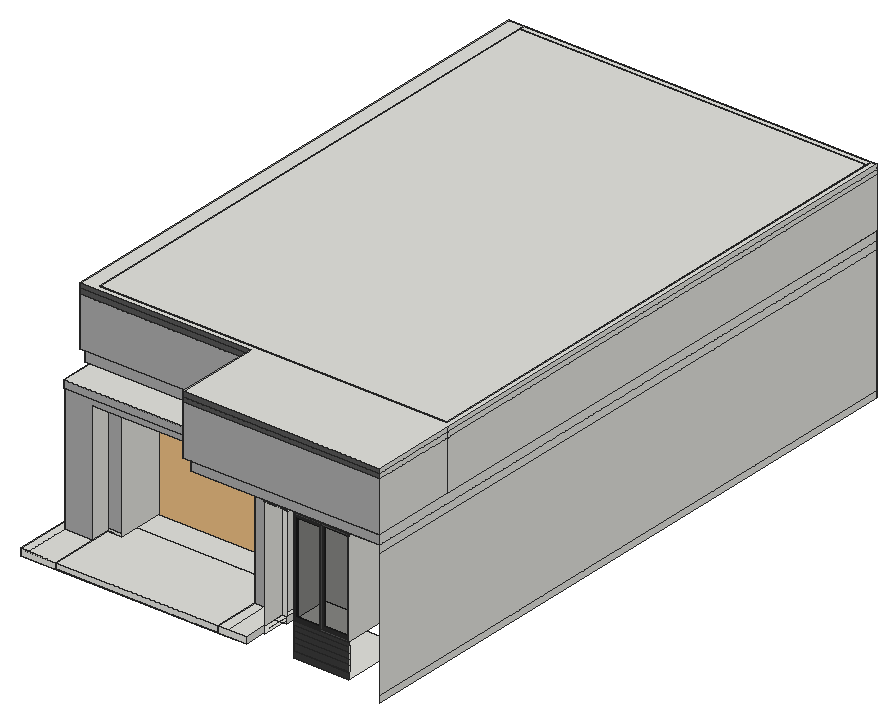
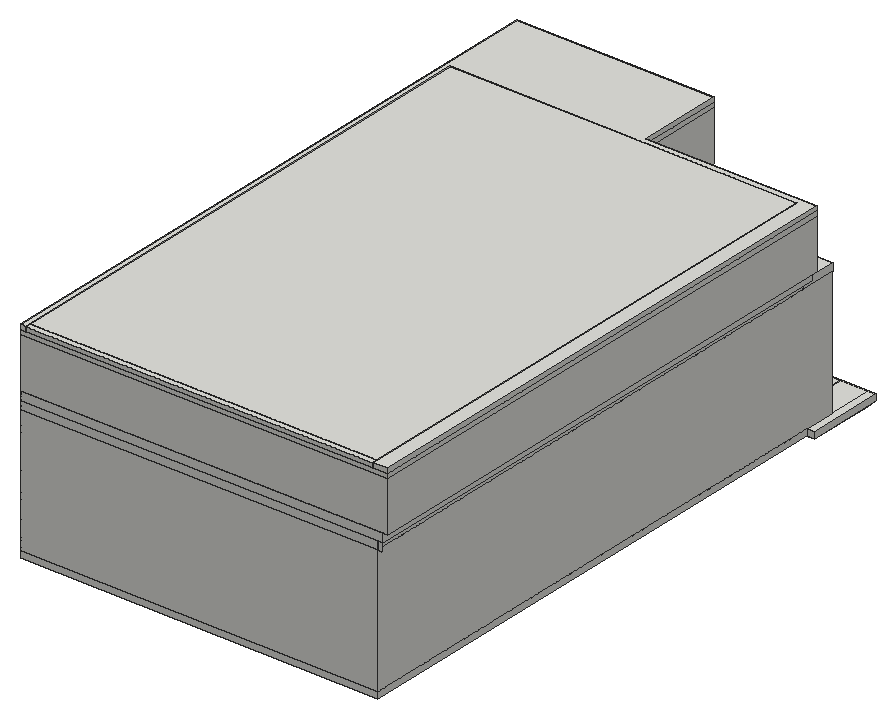
# SketchUp Ruby script. Lengths in inches.
U = 1.inch
M = Sketchup.active_model
def pt(a) = Geom::Point3d.new(a.map { |v| v * U })
def face(e, loops, mat)
  f = e.add_face(loops[0].map { |a| pt(a) })
  loops[1..].each { |l| e.add_face(l.map { |a| pt(a) }).erase! }
  f.material = f.back_material = mat if mat
  f
end
# faces: each face lists its corners as indices into pts; further lists are holes
def faces(e, pts, list, mat = nil) = list.each { |f| face(e, (f[0].is_a?(Array) ? f : [f]).map { |l| l.map { |i| pts[i] } }, mat) }
# xy, xz, yz: faces in a plane at the given z, y or x. An outline is a flat list of corners, or four numbers for a rectangle; further outlines are holes
def ring(l) = l.size == 4 ? [[l[0], l[1]], [l[2], l[1]], [l[2], l[3]], [l[0], l[3]]] : l.each_slice(2).to_a
def flat(e, list, mat, &to3) = list.each { |f| face(e, (f[0].is_a?(Array) ? f : [f]).map { |l| ring(l).map { |u, v| to3.(u, v) } }, mat) }
def xy(e, z, list, mat = nil) = flat(e, list, mat) { |x, y| [x, y, z] }
def xz(e, y, list, mat = nil) = flat(e, list, mat) { |x, z| [x, y, z] }
def yz(e, x, list, mat = nil) = flat(e, list, mat) { |y, z| [x, y, z] }
def lines(e, pts, list) = list.each { |a, b| e.add_line(pt(pts[a]), pt(pts[b])) }
# prism: a flat outline (further loops are holes) pulled along v
def prism(e, loops, v, mat = nil)
  f = face(e, loops, mat); d = Geom::Vector3d.new(v.map { |x| x * U })
  f.pushpull(f.normal.samedirection?(d) ? d.length : -d.length)
end
def box(e, o, s, mat = nil) = prism(e, [[o, [o[0] + s[0], o[1], o[2]], [o[0] + s[0], o[1] + s[1], o[2]], [o[0], o[1] + s[1], o[2]]]], [0, 0, s[2]], mat)
def at(x, y, z, deg = 0) = Geom::Transformation.translation(pt([x, y, z])) * Geom::Transformation.rotation(ORIGIN, Z_AXIS, deg.degrees)
def axes(o, x, y, z) = Geom::Transformation.new([*x, 0, *y, 0, *z, 0, *pt(o).to_a, 1])
def part(name) = M.definitions.add(name)
# library, detail: a bought-in or finely detailed component or shape, given as its bounding box
def library(name, o, s) = part(name).tap { |d| box(d.entities, o, s) }
def detail(e, o, s) = box(e.add_group.entities, o, s)
def put(e, d, t, mat = nil) = e.add_instance(d, t).tap { |i| i.material = mat if mat }
def group(e, t, mat = nil) = e.add_group.tap { |g| g.transformation = t; g.material = mat if mat }.entities
root = M.entities
M.materials.add("Glass_Tinted_Gray").color = [0, 0, 0]
M.materials["Glass_Tinted_Gray"].alpha = 0.125
M.materials.add("[0135_DarkGray]").color = [81, 81, 81]
M.materials.add("[Color M03]").color = [170, 170, 170]
M.materials.add("[Color M06]").color = [86, 86, 86]
M.materials.add("[Color M07]").color = [58, 58, 58]
M.materials.add("[Mirror 02]").color = [229, 229, 229]
M.materials.add("[Terrazzo Light Blue]").color = [196, 214, 227]
c1 = library("12",[112.18,111.43,0],[146.07,15.17,104.72])
c2 = part("PENTEK_RP Fineline 50S_Sliding_DoorCase_E1")
box(c2.entities,[0,0,0],[1.51,3.66,99.27],"[0135_DarkGray]")
c3 = part("PENTEK_RP Fineline 50S_SlidingDooe_Case_E2")
box(c3.entities,[0,0,0],[96.25,3.66,1.51],"[0135_DarkGray]")
c4 = part("pentek_RP Fineline 50S_SlidingDoor_Case")
put(c4.entities,c2,at(97.76,0,0))
put(c4.entities,c3,at(1.51,0,0))
put(c4.entities,c2,at(0,0,0))
put(c4.entities,c3,at(1.51,0,97.76))
c5 = part("PENTEK_RP Fineline 50S_SlidingDoor_GlazingBead_2")
box(c5.entities,[0,0,0],[0.56,0.59,94.39],"[0135_DarkGray]")
c6 = part("PENTEK_RP Fineline 50S_SlidingDoor_Glass")
box(c6.entities,[0,0,0],[46.58,0.16,94.39],"Glass_Tinted_Gray")
c7 = part("PENTEK_RP Fineline 50S_SlidingDoor_GlazingBead")
box(c7.entities,[0,0,0],[45.47,0.59,0.56],"[0135_DarkGray]")
c8 = part("PENTEK_RP Fineline 50S_SlidingDoor_Leaf_E1")
xy(c8.entities,0,[[0,0,0.93,1.97],[0.93,1.57,1.49,1.97]],"[0135_DarkGray]")
xy(c8.entities,96.25,[[0,0,0.93,0,0.93,1.57,1.49,1.57,1.49,1.97,0,1.97]],"[0135_DarkGray]")
xz(c8.entities,0,[[0,0,0.93,96.25]],"[0135_DarkGray]")
xz(c8.entities,1.57,[[0.93,0,1.49,95.32],[0.93,95.32,1.49,96.25]],"[0135_DarkGray]")
xz(c8.entities,1.97,[[0,0,1.49,96.25]],"[0135_DarkGray]")
yz(c8.entities,0,[[0,0,1.97,96.25]],"[0135_DarkGray]")
yz(c8.entities,0.93,[[0,0,1.57,0.93],[0,0.93,1.57,95.32],[0,95.32,1.57,96.25]],"[0135_DarkGray]")
yz(c8.entities,1.49,[[1.57,0,1.97,95.32],[1.57,95.32,1.97,96.25]],"[0135_DarkGray]")
c9 = part("PENTEK_RP Fineline 50S_SlidingDoor_Leaf_E2")
xy(c9.entities,0,[[0,0,0,1.57,0.56,1.57,0.56,1.97,46.02,1.97,46.02,1.57,46.58,1.57,46.58,0]],"[0135_DarkGray]")
xy(c9.entities,0.93,[[0,0,46.58,1.57]],"[0135_DarkGray]")
xy(c9.entities,1.49,[[0.56,1.57,46.02,1.97]],"[0135_DarkGray]")
xz(c9.entities,0,[[0,0,46.58,0.93]],"[0135_DarkGray]")
xz(c9.entities,1.57,[[0,0,0.56,0.93],[46.02,0,46.58,0.93],[0.56,0.93,46.02,1.49]],"[0135_DarkGray]")
xz(c9.entities,1.97,[[0.56,0,46.02,1.49]],"[0135_DarkGray]")
yz(c9.entities,0,[[0,0,1.57,0.93]],"[0135_DarkGray]")
yz(c9.entities,0.56,[[1.57,0,1.97,0.93],[1.57,0.93,1.97,1.49]],"[0135_DarkGray]")
yz(c9.entities,46.02,[[1.57,0,1.97,0.93],[1.57,0.93,1.97,1.49]],"[0135_DarkGray]")
yz(c9.entities,46.58,[[0,0,1.57,0.93]],"[0135_DarkGray]")
c10 = part("PENTEK_RP Fineline S_SlidingDoor_Leaf1")
put(c10.entities,c5,at(0.93,0,0.93))
put(c10.entities,c5,at(46.96,0,0.93))
put(c10.entities,c6,at(1.49,1.42,0.93))
put(c10.entities,c7,at(1.49,0,0.93))
put(c10.entities,c6,at(1.49,0.59,0.93),"[Terrazzo Light Blue]")
put(c10.entities,c8,at(0,0,0))
put(c10.entities,c8,axes([48.44,0,0],[-1,0,0],[0,1,0],[0,0,1]))
put(c10.entities,c9,axes([0.93,0,96.25],[1,0,0],[0,1,0],[0,0,-1]))
put(c10.entities,c9,at(0.93,0,0))
put(c10.entities,c7,at(1.49,0,94.77))
c11 = part("PENTEK_RP Fineline 50S_SlidingDoor_Leaf2")
put(c11.entities,c6,at(1.49,1.42,0.93))
put(c11.entities,c7,at(1.49,0,94.77))
put(c11.entities,c5,at(46.96,0,0.93))
put(c11.entities,c6,at(1.49,0.59,0.93),"[Mirror 02]")
put(c11.entities,c5,at(0.93,0,0.93))
put(c11.entities,c8,at(0,0,0))
put(c11.entities,c8,axes([48.44,0,0],[-1,0,0],[0,1,0],[0,0,1]))
put(c11.entities,c7,at(1.49,0,0.93))
put(c11.entities,c9,axes([0.93,0,96.25],[1,0,0],[0,1,0],[0,0,-1]))
put(c11.entities,c9,at(0.93,0,0))
c12 = part("PENTEK - Slimmest Steel Sliding Door / Window\#1")
put(c12.entities,c4,at(0,-1.88,-0.09))
put(c12.entities,c10,at(1.51,-2.27,1.42))
put(c12.entities,c11,at(49.32,-0.3,1.42))
c13 = library("Group\#72",[-0.5,-0.5,0],[113.04,13,1.125])
xy(root,246,[[184.16,507.49,380.7,517.74],[380.7,507.49,398.6,517.74],[184.16,517.74,189.35,580.49],[365.35,517.74,390.22,517.74,390.22,549.55,399.1,549.55,399.1,580.49,365.35,580.49],[390.22,517.74,398.6,517.74,398.6,528.52,399.1,528.52,399.1,549.55,390.22,549.55],
  [399.1,549.55,402.91,585.58],[365.35,580.49,399.1,585.58],[365.35,585.58,399.1,634.36]])
xy(root,246.1875,[[218.17,507.49,218.17,568.22,223.86,568.22,223.86,585.58,362.1,585.58,362.1,568.22,371.29,568.22,371.29,507.49]])
xy(root,246.25,[[439.12,512.52,491.67,577.96]])
xy(root,252,[[184.16,507.49,191.6,580.49],[191.6,507.49,218.17,550.86],[218.17,507.49,371.29,507.49,371.29,568.22,362.1,568.22,362.1,585.58,232.11,585.58,232.11,568.22,218.17,568.22],[371.29,507.49,380.7,550.86],[380.7,507.49,398.6,550.86],
  [398.6,528.52,398.66,549.55],[398.6,549.55,402.91,585.58],[371.29,550.86,380.7,631.58],[380.7,550.86,398.6,631.58],[223.86,568.22,232.11,585.58],
  [232.11,585.58,362.1,585.58,362.1,631.58,371.29,631.58,371.29,633.05,398.6,633.05,398.6,585.58,525.63,585.58,525.63,1083.4,196.6875,1083.4,196.6875,631.58,217.86,631.58,217.86,746.45,223.86,746.45,223.86,631.58,232.11,631.58],[217.86,631.58,223.86,746.45],[371.29,631.58,380.7,633.05],[380.7,631.58,398.6,633.05]])
xy(root,252.37,[[439.12,512.52,491.67,513.21]])
xy(root,274.3125,[[439.12,512.52,491.67,513.21]])
xy(root,278.25,[[439.12,512.52,491.67,549.55]])
xy(root,365.8125,[[[218.17,550.86,218.17,568.22,232.11,568.22,232.11,631.58,362.1,631.58,362.1,568.22,371.29,568.22,371.29,550.86],[347.6,562.2,349.15,562.4,350.6,563,351.84,563.96,352.79,565.2,353.39,566.65,353.6,568.2,353.39,569.75,352.79,571.2,351.84,572.44,350.6,573.4,349.15,574,347.6,574.2,346.04,574,344.6,573.4,343.35,572.44,342.4,571.2,341.8,569.75,341.6,568.2,341.8,566.65,342.4,565.2,343.35,563.96,344.6,563,346.04,562.4],[247.56,562.2,249.11,562.4,250.56,563,251.8,563.96,252.75,565.2,253.35,566.65,253.56,568.2,253.35,569.75,252.75,571.2,251.8,572.44,250.56,573.4,249.11,574,247.56,574.2,246,574,244.56,573.4,243.31,572.44,242.36,571.2,241.76,569.75,241.56,568.2,241.76,566.65,242.36,565.2,243.31,563.96,244.56,563,246,562.4],[299.84,562.2,301.39,562.4,302.84,563,304.08,563.96,305.04,565.2,305.64,566.65,305.84,568.2,305.64,569.75,305.04,571.2,304.08,572.44,302.84,573.4,301.39,574,299.84,574.2,298.29,574,296.84,573.4,295.6,572.44,294.64,571.2,294.04,569.75,293.84,568.2,294.04,566.65,294.64,565.2,295.6,563.96,296.84,563,298.29,562.4]],[362.1,568.22,371.29,585.58]])
xy(root,369.375,[[410.48,512.52,415.12,513.21],[415.12,512.52,416.48,528.52],[416.48,512.52,421.12,513.21],[421.12,512.52,422.48,528.52],[422.48,512.52,427.12,513.21],
  [427.12,512.52,428.48,528.52],[428.48,512.52,433.12,513.21],[433.12,512.52,434.48,528.52],[439.12,512.52,491.67,549.55]])
xy(root,372,[[191.6,549.55,398.6,550.86],[191.6,550.86,398.6,585.58],[196.6875,585.58,398.6,631.58]])
xy(root,375.375,[[410.48,512.52,497.28,528.52]])
xy(root,379.5625,[[515.78,500.24,515.78,580.49,501.41,580.49,501.41,585.58,525.63,585.58,525.63,1083.4,196.6875,1083.4,196.6875,585.58,191.6,585.58,191.6,1088.49,530.72,1088.49,530.72,500.24],[351.11,500.24,351.11,549.55,398.66,549.55,398.66,528.52,508.41,528.52,508.41,505.61,501.41,505.61,501.41,500.24],[501.41,500.24,501.41,505.61,513.53,505.61,513.53,502.86,508.41,502.86,508.41,500.24],[508.41,500.24,515.78,502.86],[513.53,502.86,513.53,521.24,508.41,521.24,508.41,580.49,515.78,580.49,515.78,502.86],
  [508.41,505.61,513.53,521.24],[398.66,528.52,402.91,549.55],[402.91,528.52,501.41,549.55],[501.41,528.52,508.41,580.49],[191.6,549.55,351.11,580.49],
  [351.11,549.55,501.41,585.58],[186.66,580.49,187.78,1088.49],[187.78,580.49,191.6,1088.49],[191.6,580.49,351.11,585.58]])
xy(root,388.5625,[[344.29,500.24,351.11,507.49],[351.11,500.24,530.72,580.49],[344.29,507.49,351.11,580.49],[182.47,580.49,186.66,1088.49],[[186.66,580.49,530.72,1088.49],[196.6875,585.58,525.63,1083.4]]])
xy(root,435.5,[[[344.29,500.24,344.29,580.49,182.47,580.49,182.47,1088.49,530.72,1088.49,530.72,500.24],[196.6875,585.58,525.63,1083.4]]])
xy(root,440.1875,[[344.29,500.24,344.29,580.49,182.47,580.49,182.47,1088.49,196.6875,1088.49,196.6875,585.58,525.63,585.58,525.63,1088.49,530.72,1088.49,530.72,500.24],[196.6875,585.58,525.63,1083.4],[196.6875,1083.4,525.63,1088.49]])
xy(root,444.75,[[344.29,500.24,530.72,500.24,530.72,1088.49,525.63,1088.49,525.63,585.58,196.6875,585.58,196.6875,1088.49,182.47,1088.49,182.47,580.49,344.29,580.49],[196.6875,585.58,525.63,1083.4],[196.6875,1083.4,525.63,1088.49]])
xz(root,500.24,[[351.11,379.5625,530.72,388.5625],[344.29,388.5625,530.72,435.5]],"[Color M03]")
xz(root,500.24,[[344.29,435.5,530.72,440.1875],[344.29,440.1875,530.72,444.75]],"[Color M06]")
xz(root,507.49,[[184.16,246,398.6,246,398.6,252,371.29,252,371.29,246.1875,218.17,246.1875,218.17,252,184.16,252],[218.17,246.1875,371.29,252]])
xz(root,512.52,[[439.12,246.25,491.67,252.37],[439.12,274.3125,491.67,278.25]],"[Color M07]")
xz(root,513.21,[[439.12,252.37,491.67,258.48],[439.12,258.48,491.67,263.48],[439.12,263.48,491.67,269.03],[439.12,269.03,491.67,274.3125]],"[Color M07]")
xz(root,549.55,[[398.66,252,402.91,379.5625]])
xz(root,549.55,[[398.6,252,398.66,252,398.66,379.5625,191.6,379.5625,191.6,372,398.6,372]],"[Color M03]")
xz(root,550.86,[[191.6,252,218.17,252,218.17,365.8125,371.29,365.8125,371.29,252,398.6,252,398.6,372,191.6,372]],"[Color M03]")
xz(root,568.22,[[218.17,246.1875,223.86,252],[362.1,246.1875,371.29,252],[218.17,252,232.11,254.6875]])
xz(root,568.22,[[362.1,252,371.29,365.8125],[218.17,254.6875,232.11,365.8125]],"[Color M03]")
xz(root,580.49,[[184.16,246,191.6,252]])
xz(root,580.49,[[186.66,379.5625,351.11,388.5625],[182.47,388.5625,344.29,435.5]],"[Color M03]")
xz(root,580.49,[[182.47,435.5,344.29,440.1875],[182.47,440.1875,344.29,444.75]],"[Color M06]")
xz(root,585.58,[[223.86,246.1875,362.1,252],[398.6,252,501.41,372],[501.41,252,525.63,372],[191.6,372,196.6875,379.5625],[196.6875,372,501.41,379.5625],
  [501.41,372,525.63,379.5625],[196.6875,379.5625,525.63,388.5625],[196.6875,388.5625,525.63,435.5],[196.6875,435.5,525.63,440.1875],[196.6875,440.1875,525.63,444.75]])
xz(root,631.58,[[196.6875,252,196.6875,372,398.6,372,398.6,252,362.1,252,362.1,365.8125,232.11,365.8125,232.11,252]])
xz(root,633.05,[[371.29,252,398.6,365.8125]])
xz(root,1083.4,[[196.6875,252,525.63,372],[196.6875,372,525.63,379.5625],[196.6875,379.5625,525.63,388.5625],[196.6875,388.5625,525.63,435.5],[196.6875,435.5,525.63,440.1875],
  [196.6875,440.1875,525.63,444.75]])
xz(root,1088.49,[[191.6,246,530.72,252],[191.6,252,530.72,372],[187.78,372,191.6,379.5625],[191.6,372,530.72,379.5625],[186.66,379.5625,530.72,388.5625],
  [182.47,388.5625,530.72,435.5],[182.47,435.5,530.72,440.1875],[182.47,440.1875,196.6875,444.75],[196.6875,440.1875,525.63,444.75],[525.63,440.1875,530.72,444.75]])
yz(root,182.47,[[580.49,388.5625,1088.49,435.5],[580.49,435.5,1088.49,440.1875],[580.49,440.1875,1088.49,444.75]])
yz(root,184.16,[[507.49,246,580.49,252]])
yz(root,186.66,[[580.49,379.5625,1088.49,388.5625]])
yz(root,191.6,[[580.49,246,1088.49,252],[550.86,252,1088.49,372],[549.55,372,585.58,379.5625],[585.58,372,1088.49,379.5625]])
yz(root,196.6875,[[631.58,252,1083.4,372],[585.58,372,1083.4,379.5625],[585.58,379.5625,1083.4,388.5625],[585.58,388.5625,1083.4,435.5],[585.58,435.5,1083.4,440.1875],
  [585.58,440.1875,1083.4,444.75],[1083.4,440.1875,1088.49,444.75]])
yz(root,218.17,[[507.49,246.1875,550.86,252],[550.86,246.1875,568.22,252],[550.86,252,568.22,365.8125]])
yz(root,223.86,[[568.22,246.1875,585.58,252]])
yz(root,232.11,[[568.22,252,631.58,365.8125]])
yz(root,344.29,[[500.24,388.5625,580.49,435.5],[500.24,435.5,580.49,440.1875],[500.24,440.1875,580.49,444.75]])
yz(root,351.11,[[500.24,379.5625,580.49,388.5625]])
yz(root,362.1,[[568.22,246.1875,585.58,252],[568.22,252,631.58,365.8125]])
yz(root,371.29,[[507.49,246.1875,550.86,252],[550.86,246.1875,568.22,252],[550.86,252,568.22,365.8125],[568.22,252,633.05,365.8125]])
yz(root,398.6,[[507.49,246,528.52,252],[549.55,252,550.86,365.8125],[550.86,252,585.58,365.8125],[585.58,252,631.58,365.8125],[631.58,252,633.05,365.8125],
  [549.55,365.8125,550.86,372],[550.86,365.8125,585.58,372],[585.58,365.8125,631.58,372]])
yz(root,398.66,[[528.52,252,549.55,379.5625]])
yz(root,402.91,[[549.55,246,585.58,252]])
yz(root,410.48,[[512.52,369.375,528.52,375.375]])
yz(root,439.12,[[512.52,252.37,513.21,258.48],[512.52,258.48,513.21,263.48],[512.52,263.48,513.21,269.03],[512.52,269.03,513.21,274.3125],[512.52,278.25,549.55,369.375]])
yz(root,491.67,[[512.52,252.37,513.21,258.48],[512.52,258.48,513.21,263.48],[512.52,263.48,513.21,269.03],[512.52,269.03,513.21,274.3125],[512.52,278.25,549.55,369.375]])
yz(root,525.63,[[585.58,252,1083.4,372],[585.58,372,1083.4,379.5625],[585.58,379.5625,1083.4,388.5625],[585.58,388.5625,1083.4,435.5],[585.58,435.5,1083.4,440.1875],
  [585.58,440.1875,1083.4,444.75],[1083.4,440.1875,1088.49,444.75]])
yz(root,530.72,[[500.24,246,1088.49,252],[500.24,252,1088.49,372],[500.24,372,1088.49,379.5625],[500.24,379.5625,1088.49,388.5625],[500.24,388.5625,580.49,435.5],
  [580.49,388.5625,1088.49,435.5],[500.24,435.5,580.49,440.1875],[580.49,435.5,1088.49,440.1875],[500.24,440.1875,580.49,444.75],[580.49,440.1875,1088.49,444.75]])
p = [[247.56,562.2,365.8125],[246,562.4,365.8125],[246,562.4,367.875],[247.56,562.2,367.875],[249.11,562.4,365.8125],[249.11,562.4,367.875],
  [299.84,562.2,365.8125],[298.29,562.4,365.8125],[298.29,562.4,367.625],[299.84,562.2,367.625],[301.39,562.4,365.8125],[301.39,562.4,367.625],
  [347.6,562.2,365.8125],[346.04,562.4,365.8125],[346.04,562.4,366.75],[347.6,562.2,366.75],[349.15,562.4,365.8125],[349.15,562.4,366.75],
  [244.56,563,365.8125],[244.56,563,367.875],[250.56,563,365.8125],[250.56,563,367.875],[296.84,563,365.8125],[296.84,563,367.625],
  [302.84,563,365.8125],[302.84,563,367.625],[344.6,563,365.8125],[344.6,563,366.75],[350.6,563,365.8125],[350.6,563,366.75],
  [243.31,563.96,365.8125],[243.31,563.96,367.875],[251.8,563.96,365.8125],[251.8,563.96,367.875],[295.6,563.96,365.8125],[295.6,563.96,367.625],
  [304.08,563.96,365.8125],[304.08,563.96,367.625],[343.35,563.96,365.8125],[343.35,563.96,366.75],[351.84,563.96,365.8125],[351.84,563.96,366.75],
  [242.36,565.2,365.8125],[242.36,565.2,367.875],[252.75,565.2,365.8125],[252.75,565.2,367.875],[294.64,565.2,365.8125],[294.64,565.2,367.625],
  [305.04,565.2,365.8125],[305.04,565.2,367.625],[342.4,565.2,365.8125],[342.4,565.2,366.75],[352.79,565.2,365.8125],[352.79,565.2,366.75],
  [241.76,566.65,365.8125],[241.76,566.65,367.875],[253.35,566.65,365.8125],[253.35,566.65,367.875],[294.04,566.65,365.8125],[294.04,566.65,367.625],
  [305.64,566.65,365.8125],[305.64,566.65,367.625],[341.8,566.65,365.8125],[341.8,566.65,366.75],[353.39,566.65,365.8125],[353.39,566.65,366.75],
  [241.56,568.2,365.8125],[241.56,568.2,367.875],[253.56,568.2,365.8125],[253.56,568.2,367.875],[293.84,568.2,365.8125],[293.84,568.2,367.625],
  [305.84,568.2,365.8125],[305.84,568.2,367.625],[341.6,568.2,365.8125],[341.6,568.2,366.75],[353.6,568.2,365.8125],[353.6,568.2,366.75],
  [241.76,569.75,365.8125],[241.76,569.75,367.875],[253.35,569.75,365.8125],[253.35,569.75,367.875],[294.04,569.75,365.8125],[294.04,569.75,367.625],
  [305.64,569.75,365.8125],[305.64,569.75,367.625],[341.8,569.75,365.8125],[341.8,569.75,366.75],[353.39,569.75,365.8125],[353.39,569.75,366.75],
  [242.36,571.2,365.8125],[242.36,571.2,367.875],[252.75,571.2,365.8125],[252.75,571.2,367.875],[294.64,571.2,365.8125],[294.64,571.2,367.625],
  [305.04,571.2,365.8125],[305.04,571.2,367.625],[342.4,571.2,365.8125],[342.4,571.2,366.75],[352.79,571.2,365.8125],[352.79,571.2,366.75],
  [243.31,572.44,365.8125],[243.31,572.44,367.875],[251.8,572.44,365.8125],[251.8,572.44,367.875],[295.6,572.44,365.8125],[295.6,572.44,367.625],
  [304.08,572.44,365.8125],[304.08,572.44,367.625],[343.35,572.44,365.8125],[343.35,572.44,366.75],[351.84,572.44,365.8125],[351.84,572.44,366.75],
  [244.56,573.4,365.8125],[244.56,573.4,367.875],[250.56,573.4,365.8125],[250.56,573.4,367.875],[296.84,573.4,365.8125],[296.84,573.4,367.625],
  [302.84,573.4,365.8125],[302.84,573.4,367.625],[344.6,573.4,365.8125],[344.6,573.4,366.75],[350.6,573.4,365.8125],[350.6,573.4,366.75],
  [246,574,365.8125],[246,574,367.875],[249.11,574,365.8125],[249.11,574,367.875],[298.29,574,365.8125],[298.29,574,367.625],
  [301.39,574,365.8125],[301.39,574,367.625],[346.04,574,365.8125],[346.04,574,366.75],[349.15,574,365.8125],[349.15,574,366.75],
  [247.56,574.2,365.8125],[247.56,574.2,367.875],[299.84,574.2,365.8125],[299.84,574.2,367.625],[347.6,574.2,365.8125],[347.6,574.2,366.75],
  [402.91,549.55,252],[402.91,528.52,252],[371.29,585.58,365.8125],[373.1,585.58,365.8125]]
faces(root,p,[[0,1,2,3],[4,0,3,5],[6,7,8,9],[10,6,9,11],[12,13,14,15],[16,12,15,17],[1,18,19,2],[20,4,5,21],
  [7,22,23,8],[24,10,11,25],[13,26,27,14],[28,16,17,29],[18,30,31,19],[32,20,21,33],[22,34,35,23],[36,24,25,37],
  [26,38,39,27],[40,28,29,41],[30,42,43,31],[44,32,33,45],[34,46,47,35],[48,36,37,49],[38,50,51,39],[52,40,41,53],
  [42,54,55,43],[56,44,45,57],[46,58,59,47],[60,48,49,61],[50,62,63,51],[64,52,53,65],[54,66,67,55],[68,56,57,69],
  [58,70,71,59],[72,60,61,73],[62,74,75,63],[76,64,65,77],[66,78,79,67],[80,68,69,81],[70,82,83,71],[84,72,73,85],
  [74,86,87,75],[88,76,77,89],[78,90,91,79],[92,80,81,93],[82,94,95,83],[96,84,85,97],[86,98,99,87],[100,88,89,101],
  [90,102,103,91],[104,92,93,105],[94,106,107,95],[108,96,97,109],[98,110,111,99],[112,100,101,113],[102,114,115,103],[116,104,105,117],
  [106,118,119,107],[120,108,109,121],[110,122,123,111],[124,112,113,125],[114,126,127,115],[128,116,117,129],[118,130,131,119],[132,120,121,133],
  [122,134,135,123],[136,124,125,137],[126,138,139,127],[138,128,129,139],[130,140,141,131],[140,132,133,141],[134,142,143,135],[142,136,137,143]])
lines(root,p,[[144,145],[146,147]])
put(root,c1,axes([68.07,476.88,245.99],[1.2096,0,0],[0,1.2096,0],[0,0,1.26831]),"[Color M06]")
put(root,c12,axes([439.12,514.4,278.33],[0.52935,0,0],[0,1,0],[0,0,0.92]))
put(root,c13,at(241.56,562.2,366.75))
